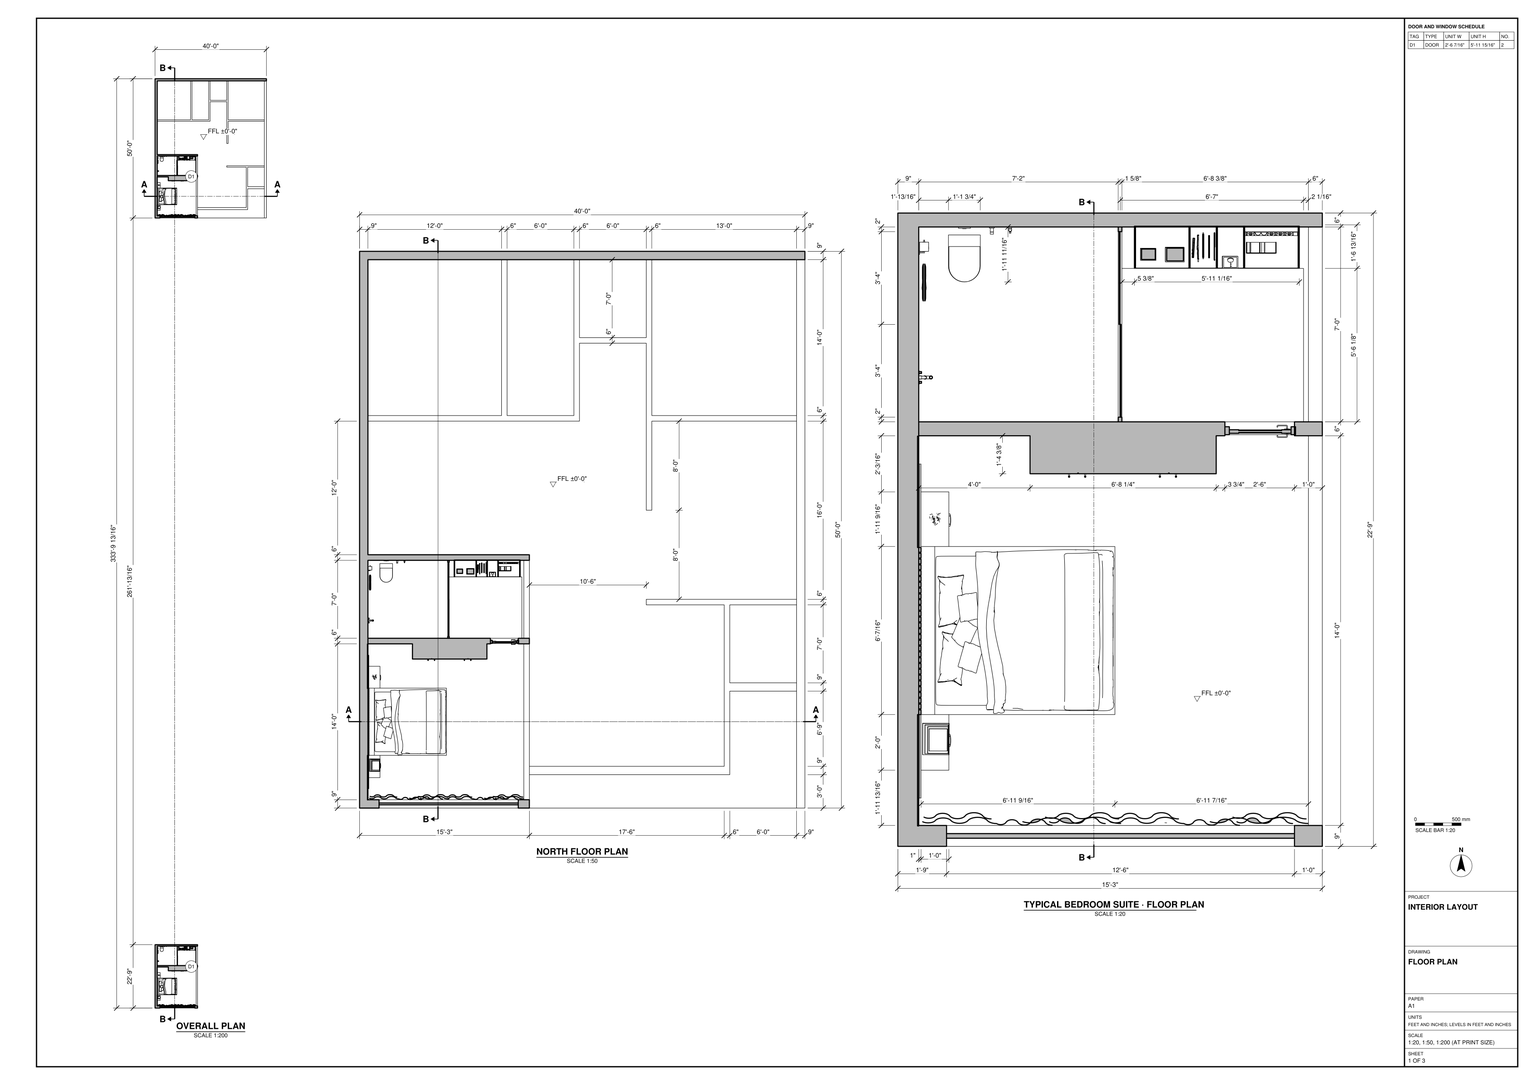
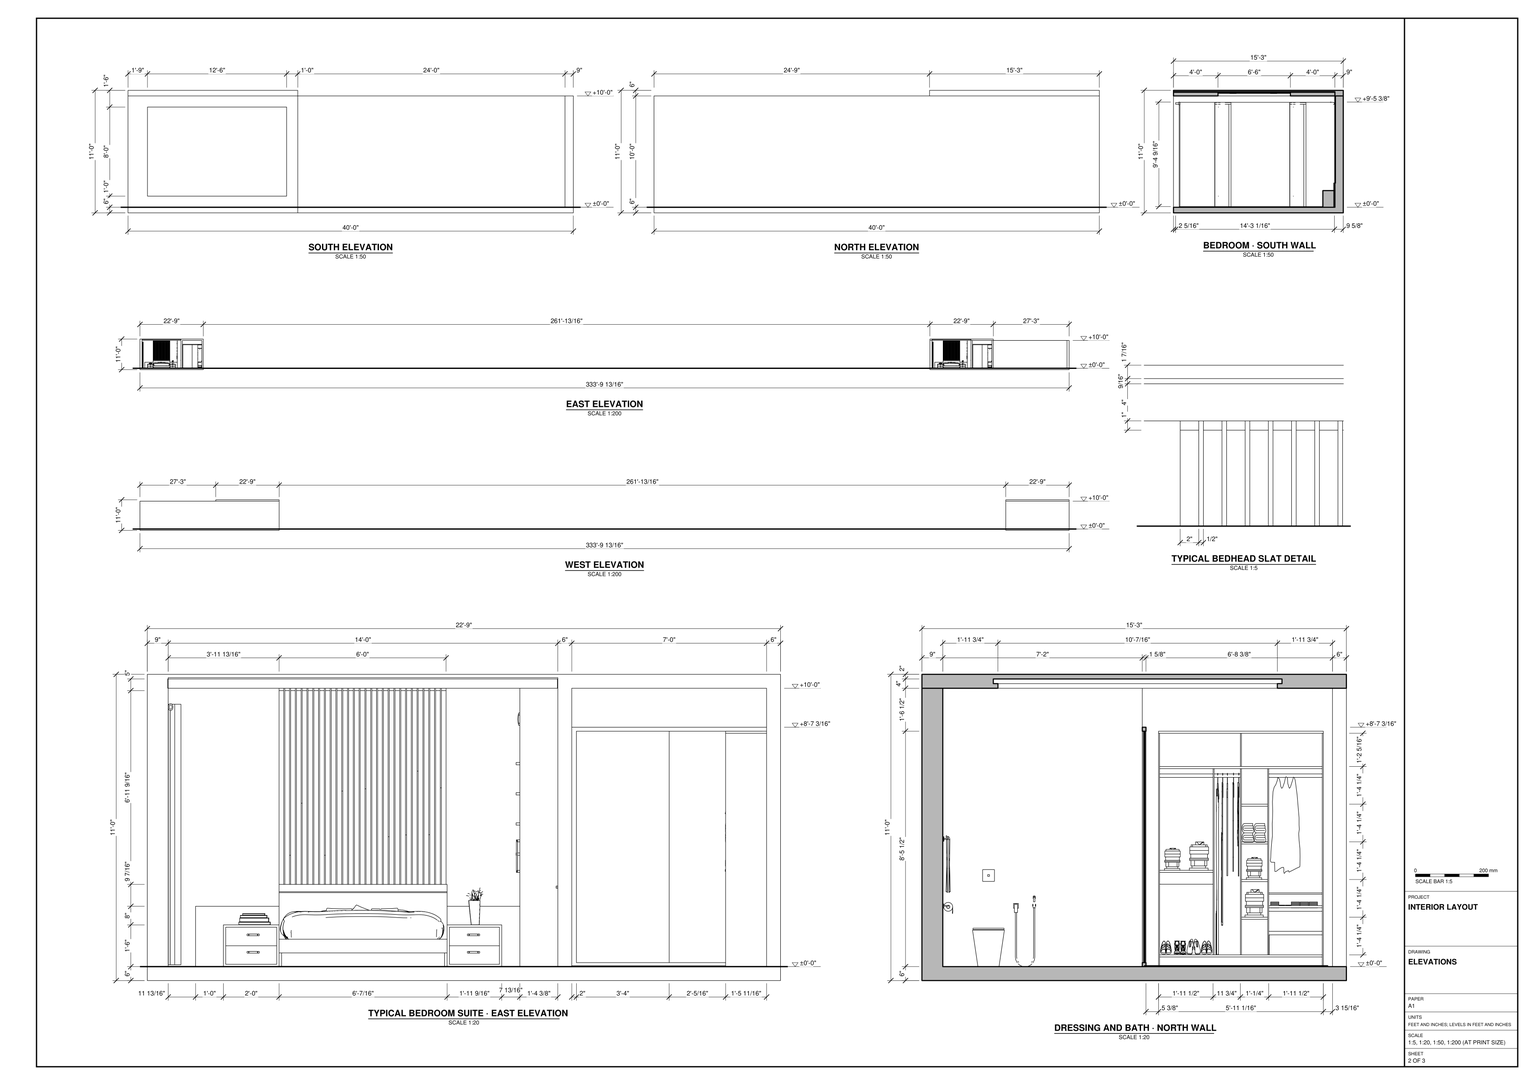
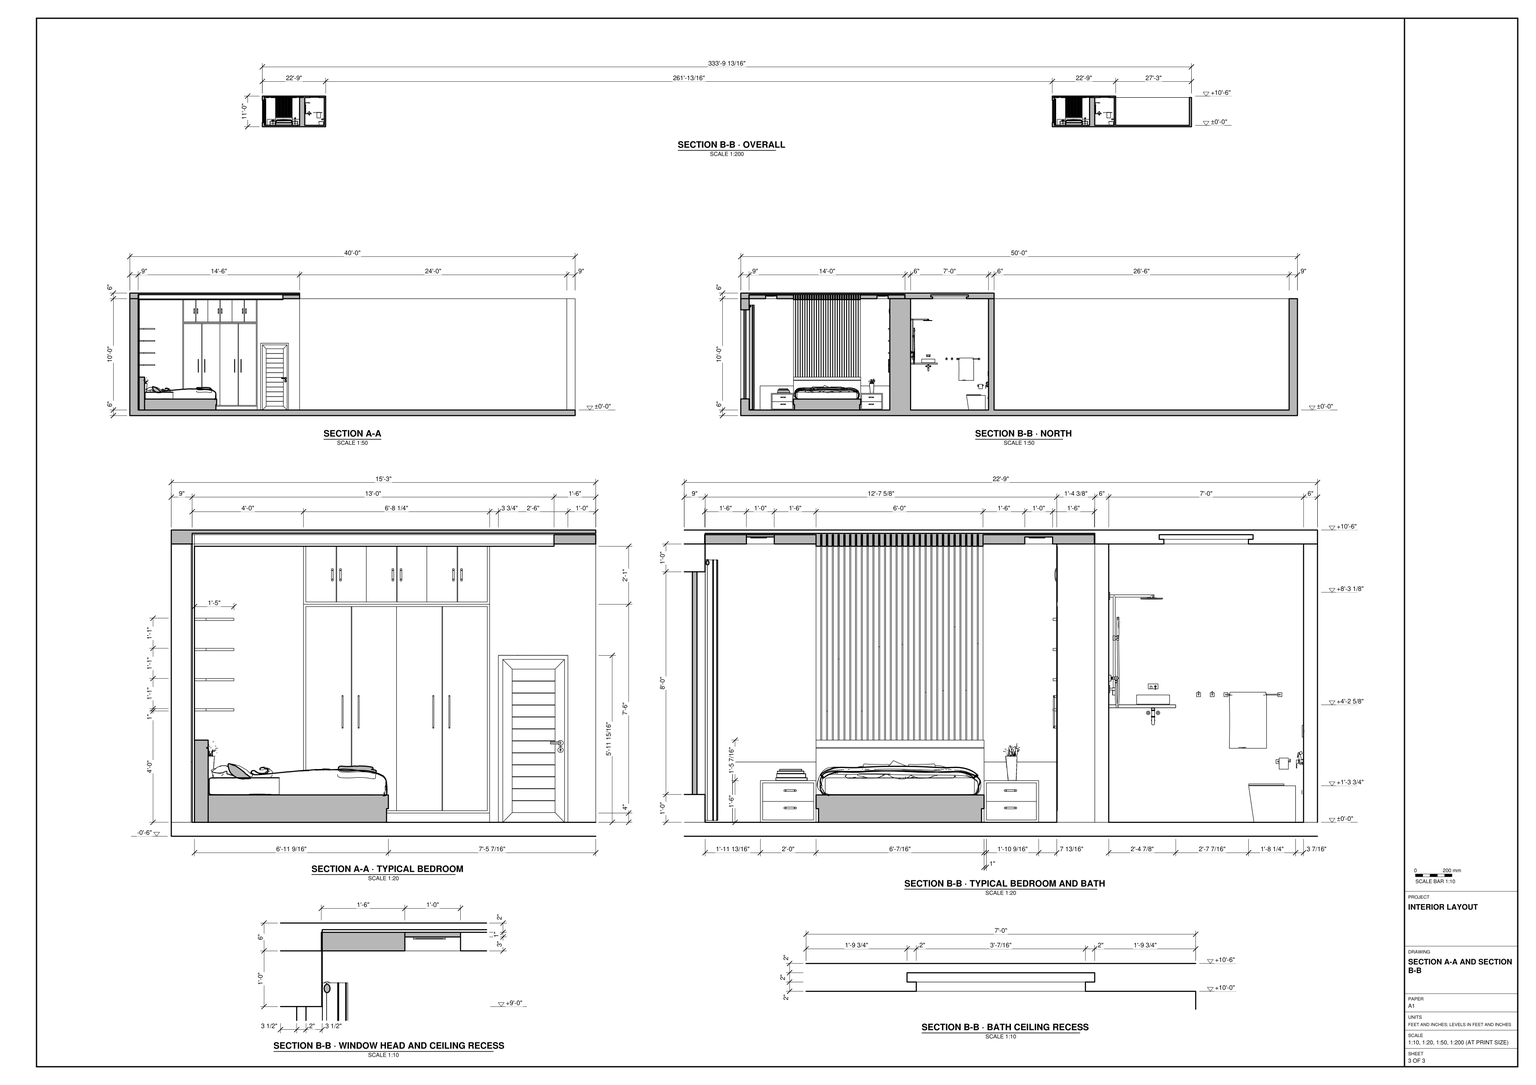
Work in feet and inches in SketchUp from task_files/diagram_01.pdf. Model the two locations shown on the overall plan: a furnished bedroom suite in the southwest corner of the 40'-0" by 50'-0" north floor layout, and a matching, separate suite to the south. Align their west walls and leave the intervening space clear. The complete model must measure 40'-0" along X, 333'-9 13/16" along Y and 11'-0" along Z. Use the single finished floor level of ±0'-0" at both locations.

Follow the north floor plan for the surrounding slab and wall layout. Use the enlarged suite plan, elevations and sections for the wall thicknesses, floor and roof slabs, ceiling recesses, bedroom window and door into the dressing area. In each suite, place the platform bed against the slatted bedhead, with a drawer unit on either side. Fit the bedroom wardrobe and overhead cupboards beside the door. Beyond the bedroom, separate the bath fixtures from the dressing bay and model the open wardrobe with its shelves, hanging spaces and drawers. Decor and loose items, including curtains, clothing, towels and plants, may be any suitable library components.

Keep shell elements such as walls, slabs and roof separate as groups or components. Group each furniture or joinery piece separately and use components for repeated parts. Save one SketchUp model as output_files/bedroom_suites_and_surrounding_north_floor_layout.skp.

# SketchUp Ruby script. Lengths in inches.
U = 1.inch
M = Sketchup.active_model
def pt(a) = Geom::Point3d.new(a.map { |v| v * U })
def face(e, loops, mat)
  f = e.add_face(loops[0].map { |a| pt(a) })
  loops[1..].each { |l| e.add_face(l.map { |a| pt(a) }).erase! }
  f.material = f.back_material = mat if mat
  f
end
# faces: each face lists its corners as indices into pts; further lists are holes
def faces(e, pts, list, mat = nil) = list.each { |f| face(e, (f[0].is_a?(Array) ? f : [f]).map { |l| l.map { |i| pts[i] } }, mat) }
# xy, xz, yz: faces in a plane at the given z, y or x. An outline is a flat list of corners, or four numbers for a rectangle; further outlines are holes
def ring(l) = l.size == 4 ? [[l[0], l[1]], [l[2], l[1]], [l[2], l[3]], [l[0], l[3]]] : l.each_slice(2).to_a
def flat(e, list, mat, &to3) = list.each { |f| face(e, (f[0].is_a?(Array) ? f : [f]).map { |l| ring(l).map { |u, v| to3.(u, v) } }, mat) }
def xy(e, z, list, mat = nil) = flat(e, list, mat) { |x, y| [x, y, z] }
def xz(e, y, list, mat = nil) = flat(e, list, mat) { |x, z| [x, y, z] }
def yz(e, x, list, mat = nil) = flat(e, list, mat) { |y, z| [x, y, z] }
def lines(e, pts, list) = list.each { |a, b| e.add_line(pt(pts[a]), pt(pts[b])) }
# prism: a flat outline (further loops are holes) pulled along v
def prism(e, loops, v, mat = nil)
  f = face(e, loops, mat); d = Geom::Vector3d.new(v.map { |x| x * U })
  f.pushpull(f.normal.samedirection?(d) ? d.length : -d.length)
end
def box(e, o, s, mat = nil) = prism(e, [[o, [o[0] + s[0], o[1], o[2]], [o[0] + s[0], o[1] + s[1], o[2]], [o[0], o[1] + s[1], o[2]]]], [0, 0, s[2]], mat)
def at(x, y, z, deg = 0) = Geom::Transformation.translation(pt([x, y, z])) * Geom::Transformation.rotation(ORIGIN, Z_AXIS, deg.degrees)
def axes(o, x, y, z) = Geom::Transformation.new([*x, 0, *y, 0, *z, 0, *pt(o).to_a, 1])
def part(name) = M.definitions.add(name)
# library, detail: a bought-in or finely detailed component or shape, given as its bounding box
def library(name, o, s) = part(name).tap { |d| box(d.entities, o, s) }
def detail(e, o, s) = box(e.add_group.entities, o, s)
def put(e, d, t, mat = nil) = e.add_instance(d, t).tap { |i| i.material = mat if mat }
def group(e, t, mat = nil) = e.add_group.tap { |g| g.transformation = t; g.material = mat if mat }.entities
root = M.entities
M.materials.add("0915 AP 7850 BANANA CREAM").color = [226, 212, 179]
M.materials.add("1833 AP 8596 CRYSTAL BEACH").color = [234, 228, 220]
M.materials.add("Carpet_Frieze_Low").color = [170, 156, 146]
M.materials.add("Carpet_Loop_Low").color = [201, 172, 127]
M.materials["Carpet_Loop_Low"].alpha = 0.3
M.materials.add("Emissive\#1").color = [251, 252, 224]
M.materials.add("Glass Bumpy 03 10cm").color = [188, 188, 188]
M.materials["Glass Bumpy 03 10cm"].alpha = 0.15
M.materials.add("Glass Safety Distorted 001").color = [249, 255, 239]
M.materials["Glass Safety Distorted 001"].alpha = 0.1
M.materials.add("Maquette Wood B01 12cm").color = [172, 139, 101]
M.materials.add("PDM_chrome").color = [38, 38, 38]
M.materials.add("Tiles Grey 13 135cm").color = [141, 141, 136]
M.materials.add("Tiles Marble White 03 180cm").color = [241, 241, 241]
M.materials.add("Tiles Patterned 07 80cm\#2").color = [154, 140, 117]
M.materials.add("W150Z669S75_Sabya 3 Gokul Pichwai-Khubanee").color = [172, 128, 96]
M.materials.add("[Aluminum]").color = [179, 179, 179]
c1 = part("Curtain panel")
p = [[17.625,0.0625,78.74],[17.625,0.0625,0],[18.27,0,0],[18.27,0,78.74],[18.92,0.0625,0],[18.92,0.0625,78.74],
  [17,0.25,78.74],[17,0.25,0],[19.55,0.25,0],[19.55,0.25,78.74],[16.43,0.56,78.74],[16.43,0.56,0],
  [20.12,0.56,0],[20.12,0.56,78.74],[6.31,0.6,78.74],[6.31,0.6,0],[6.8125,0.45,0],[6.8125,0.45,78.74],
  [7.33,0.4,0],[7.33,0.4,78.74],[7.86,0.45,0],[7.86,0.45,78.74],[8.36,0.6,0],[8.36,0.6,78.74],
  [5.85,0.85,78.74],[5.85,0.85,0],[8.82,0.85,0],[8.82,0.85,78.74],[15.92,0.97,78.74],[15.92,0.97,0],
  [20.625,0.97,0],[20.625,0.97,78.74],[5.44,1.18,78.74],[5.44,1.18,0],[9.23,1.18,0],[9.23,1.18,78.74],
  [15.51,1.48,78.74],[15.51,1.48,0],[21.04,1.48,0],[21.04,1.48,78.74],[5.11,1.59,78.74],[5.11,1.59,0],
  [9.5625,1.59,0],[9.5625,1.59,78.74],[14.93,2.55,78.74],[14.93,2.55,0],[15.2,2.04,0],[15.2,2.04,78.74],
  [21.34,2.04,0],[21.64,2.59,0],[21.64,2.59,78.74],[21.34,2.04,78.74],[4.63,2.47,78.74],[4.63,2.47,0],
  [4.86,2.04,0],[4.86,2.04,78.74],[9.81,2.04,0],[10.08,2.55,0],[10.08,2.55,78.74],[9.81,2.04,78.74],
  [4.32,2.85,78.74],[4.32,2.85,0],[10.44,2.99,0],[10.44,2.99,78.74],[14.57,2.99,78.74],[14.57,2.99,0],
  [22.03,3.0625,0],[22.03,3.0625,78.74],[0.85,2.85,78.74],[0.85,2.85,0],[1.22,3.15,0],[1.22,3.15,78.74],
  [3.95,3.15,78.74],[3.95,3.15,0],[10.89,3.35,0],[10.89,3.35,78.74],[14.125,3.35,78.74],[14.125,3.35,0],
  [22.5,3.45,0],[22.5,3.45,78.74],[1.65,3.375,0],[1.65,3.375,78.74],[3.53,3.375,78.74],[3.53,3.375,0],
  [2.11,3.52,0],[2.11,3.52,78.74],[3.07,3.52,78.74],[3.07,3.52,0],[11.39,3.625,0],[11.39,3.625,78.74],
  [13.62,3.625,78.74],[13.62,3.625,0],[2.59,3.5625,0],[2.59,3.5625,78.74],[23.04,3.74,0],[23.04,3.74,78.74],
  [11.9375,3.79,0],[11.9375,3.79,78.74],[13.07,3.79,78.74],[13.07,3.79,0],[23.63,3.92,0],[23.63,3.92,78.74],
  [12.51,3.85,0],[12.51,3.85,78.74],[24.25,3.98,0],[24.25,3.98,78.74],[5.51,1.25,0],[5.9,0.93,0],
  [4.95,2.09,0],[5.1875,1.64,0],[6.35,0.69,0],[6.83,0.55,0],[7.33,0.5,0],[7.84,0.55,0],
  [8.32,0.69,0],[8.77,0.93,0],[9.16,1.25,0],[9.48,1.64,0],[9.72,2.09,0],[10,2.61,0],
  [10.375,3.0625,0],[10.83,3.4375,0],[17.64,0.16,0],[18.27,0.1,0],[11.35,3.71,0],[11.92,3.89,0],
  [12.51,3.94,0],[13.09,3.89,0],[20.56,1.04,0],[20.96,1.53,0],[13.66,3.71,0],[14.18,3.4375,0],
  [14.64,3.0625,0],[15.01,2.61,0],[15.29,2.09,0],[15.59,1.53,0],[15.99,1.04,0],[16.48,0.64,0],
  [17.04,0.34,0],[18.9,0.16,0],[19.51,0.34,0],[20.07,0.64,0],[21.26,2.09,0],[21.56,2.64,0],
  [21.96,3.13,0],[22.45,3.53,0],[23,3.83,0],[23.61,4.01,0],[24.24,4.08,0]]
faces(c1.entities,p,[[0,1,2,3],[3,2,4,5],[6,7,1,0],[5,4,8,9],[10,11,7,6],[9,8,12,13],[14,15,16,17],[17,16,18,19],
  [19,18,20,21],[21,20,22,23],[24,25,15,14],[23,22,26,27],[28,29,11,10],[13,12,30,31],[32,33,25,24],[27,26,34,35],
  [36,37,29,28],[31,30,38,39],[40,41,33,32],[35,34,42,43],[44,45,46,37,36,47],[39,38,48,49,50,51],[52,53,54,41,40,55],[43,42,56,57,58,59],
  [60,61,53,52],[58,57,62,63],[64,65,45,44],[50,49,66,67],[68,69,70,71],[72,73,61,60],[63,62,74,75],[76,77,65,64],
  [67,66,78,79],[71,70,80,81],[82,83,73,72],[81,80,84,85],[86,87,83,82],[75,74,88,89],[90,91,77,76],[85,84,92,93],
  [93,92,87,86],[79,78,94,95],[89,88,96,97],[98,99,91,90],[95,94,100,101],[97,96,102,103],[103,102,99,98],[101,100,104,105]])
lines(c1.entities,p,[[106,107],[108,109],[109,106],[107,110],[110,111],[111,112],[112,113],[113,114],[114,115],[115,116],[116,117],[117,118],
  [118,119],[119,120],[120,121],[122,123],[121,124],[124,125],[125,126],[126,127],[128,129],[127,130],[130,131],[131,132],
  [132,133],[133,134],[134,135],[135,136],[136,137],[137,138],[138,122],[123,139],[139,140],[140,141],[141,128],[129,142],
  [142,143],[143,144],[144,145],[145,146],[146,147],[147,148],[148,104]])
c2 = part("Curtain rod section")
yz(c2.entities,0,[[1.55,0.61,1.31,0.64,1.08,0.73,0.88,0.88,0.73,1.08,0.64,1.31,0.61,1.55,0.64,1.79,0.73,2.02,0.88,2.22,1.08,2.37,1.31,2.46,1.55,2.49,1.79,2.46,2.02,2.37,2.22,2.22,2.37,2.02,2.46,1.79,2.49,1.55,2.46,1.31,2.37,1.08,2.22,0.88,2.02,0.73,1.79,0.64]])
yz(c2.entities,2.36,[[[1.55,0,1.15,0.05,0.78,0.21,0.45,0.45,0.21,0.78,0.05,1.15,0,1.55,0.05,1.95,0.21,2.33,0.45,2.65,0.78,2.89,1.15,3.05,1.55,3.1,1.95,3.05,2.33,2.89,2.65,2.65,2.89,2.33,3.05,1.95,3.1,1.55,3.05,1.15,2.89,0.78,2.65,0.45,2.33,0.21,1.95,0.05],[1.55,0.61,1.79,0.64,2.02,0.73,2.22,0.88,2.37,1.08,2.46,1.31,2.49,1.55,2.46,1.79,2.37,2.02,2.22,2.22,2.02,2.37,1.79,2.46,1.55,2.49,1.31,2.46,1.08,2.37,0.88,2.22,0.73,2.02,0.64,1.79,0.61,1.55,0.64,1.31,0.73,1.08,0.88,0.88,1.08,0.73,1.31,0.64]]])
yz(c2.entities,3.15,[[[1.55,0,1.95,0.05,2.33,0.21,2.65,0.45,2.89,0.78,3.05,1.15,3.1,1.55,3.05,1.95,2.89,2.33,2.65,2.65,2.33,2.89,1.95,3.05,1.55,3.1,1.15,3.05,0.78,2.89,0.45,2.65,0.21,2.33,0.05,1.95,0,1.55,0.05,1.15,0.21,0.78,0.45,0.45,0.78,0.21,1.15,0.05],[1.55,0.61,1.31,0.64,1.08,0.73,0.88,0.88,0.73,1.08,0.64,1.31,0.61,1.55,0.64,1.79,0.73,2.02,0.88,2.22,1.08,2.37,1.31,2.46,1.55,2.49,1.79,2.46,2.02,2.37,2.22,2.22,2.37,2.02,2.46,1.79,2.49,1.55,2.46,1.31,2.37,1.08,2.22,0.88,2.02,0.73,1.79,0.64]]])
yz(c2.entities,61.24,[[1.55,0.61,1.79,0.64,2.02,0.73,2.22,0.88,2.37,1.08,2.46,1.31,2.49,1.55,2.46,1.79,2.37,2.02,2.22,2.22,2.02,2.37,1.79,2.46,1.55,2.49,1.31,2.46,1.08,2.37,0.88,2.22,0.73,2.02,0.64,1.79,0.61,1.55,0.64,1.31,0.73,1.08,0.88,0.88,1.08,0.73,1.31,0.64]])
p = [[2.36,1.15,0.05],[2.36,1.55,0],[3.15,1.55,0],[3.15,1.15,0.05],[2.36,1.95,0.05],[3.15,1.95,0.05],
  [2.36,0.78,0.21],[3.15,0.78,0.21],[2.36,2.33,0.21],[3.15,2.33,0.21],[2.36,0.45,0.45],[3.15,0.45,0.45],
  [2.36,2.65,0.45],[3.15,2.65,0.45],[2.36,0.21,0.78],[3.15,0.21,0.78],[2.36,2.89,0.78],[3.15,2.89,0.78],
  [2.36,1.31,0.64],[2.36,1.08,0.73],[0,1.08,0.73],[0,1.31,0.64],[3.15,1.31,0.64],[3.15,1.08,0.73],
  [61.24,1.31,0.64],[61.24,1.08,0.73],[2.36,1.55,0.61],[0,1.55,0.61],[3.15,1.55,0.61],[61.24,1.55,0.61],
  [2.36,1.79,0.64],[0,1.79,0.64],[3.15,1.79,0.64],[61.24,1.79,0.64],[2.36,2.02,0.73],[0,2.02,0.73],
  [3.15,2.02,0.73],[61.24,2.02,0.73],[2.36,0.88,0.88],[0,0.88,0.88],[3.15,0.88,0.88],[61.24,0.88,0.88],
  [2.36,2.22,0.88],[0,2.22,0.88],[3.15,2.22,0.88],[61.24,2.22,0.88],[2.36,0.05,1.15],[3.15,0.05,1.15],
  [2.36,3.05,1.15],[3.15,3.05,1.15],[2.36,0.73,1.08],[0,0.73,1.08],[3.15,0.73,1.08],[61.24,0.73,1.08],
  [2.36,2.37,1.08],[0,2.37,1.08],[3.15,2.37,1.08],[61.24,2.37,1.08],[2.36,0,1.55],[3.15,0,1.55],
  [2.36,0.64,1.31],[0,0.64,1.31],[3.15,0.64,1.31],[61.24,0.64,1.31],[2.36,2.46,1.31],[0,2.46,1.31],
  [3.15,2.46,1.31],[61.24,2.46,1.31],[2.36,3.1,1.55],[3.15,3.1,1.55],[2.36,0.61,1.55],[0,0.61,1.55],
  [3.15,0.61,1.55],[61.24,0.61,1.55],[2.36,2.49,1.55],[0,2.49,1.55],[3.15,2.49,1.55],[61.24,2.49,1.55],
  [2.36,0.05,1.95],[3.15,0.05,1.95],[2.36,0.64,1.79],[0,0.64,1.79],[3.15,0.64,1.79],[61.24,0.64,1.79],
  [2.36,2.46,1.79],[0,2.46,1.79],[3.15,2.46,1.79],[61.24,2.46,1.79],[2.36,3.05,1.95],[3.15,3.05,1.95],
  [2.36,0.73,2.02],[0,0.73,2.02],[3.15,0.73,2.02],[61.24,0.73,2.02],[2.36,2.37,2.02],[0,2.37,2.02],
  [3.15,2.37,2.02],[61.24,2.37,2.02],[2.36,0.21,2.33],[3.15,0.21,2.33],[2.36,0.88,2.22],[0,0.88,2.22],
  [3.15,0.88,2.22],[61.24,0.88,2.22],[2.36,2.22,2.22],[0,2.22,2.22],[3.15,2.22,2.22],[61.24,2.22,2.22],
  [2.36,2.89,2.33],[3.15,2.89,2.33],[2.36,1.08,2.37],[0,1.08,2.37],[3.15,1.08,2.37],[61.24,1.08,2.37],
  [2.36,2.02,2.37],[0,2.02,2.37],[3.15,2.02,2.37],[61.24,2.02,2.37],[2.36,0.45,2.65],[3.15,0.45,2.65],
  [2.36,2.65,2.65],[3.15,2.65,2.65],[2.36,1.31,2.46],[0,1.31,2.46],[3.15,1.31,2.46],[61.24,1.31,2.46],
  [2.36,1.79,2.46],[0,1.79,2.46],[3.15,1.79,2.46],[61.24,1.79,2.46],[2.36,1.55,2.49],[0,1.55,2.49],
  [3.15,1.55,2.49],[61.24,1.55,2.49],[2.36,0.78,2.89],[3.15,0.78,2.89],[2.36,2.33,2.89],[3.15,2.33,2.89],
  [2.36,1.15,3.05],[3.15,1.15,3.05],[2.36,1.95,3.05],[3.15,1.95,3.05],[2.36,1.55,3.1],[3.15,1.55,3.1]]
faces(c2.entities,p,[[0,1,2,3],[1,4,5,2],[6,0,3,7],[4,8,9,5],[10,6,7,11],[8,12,13,9],[14,10,11,15],[12,16,17,13],
  [18,19,20,21],[19,18,22,23],[24,25,23,22],[26,18,21,27],[18,26,28,22],[29,24,22,28],[30,26,27,31],[26,30,32,28],
  [33,29,28,32],[34,30,31,35],[30,34,36,32],[37,33,32,36],[19,38,39,20],[38,19,23,40],[25,41,40,23],[42,34,35,43],
  [34,42,44,36],[45,37,36,44],[46,14,15,47],[16,48,49,17],[38,50,51,39],[50,38,40,52],[41,53,52,40],[54,42,43,55],
  [42,54,56,44],[57,45,44,56],[58,46,47,59],[50,60,61,51],[60,50,52,62],[53,63,62,52],[64,54,55,65],[54,64,66,56],
  [67,57,56,66],[48,68,69,49],[60,70,71,61],[70,60,62,72],[63,73,72,62],[74,64,65,75],[64,74,76,66],[77,67,66,76],
  [78,58,59,79],[70,80,81,71],[80,70,72,82],[73,83,82,72],[84,74,75,85],[74,84,86,76],[87,77,76,86],[68,88,89,69],
  [80,90,91,81],[90,80,82,92],[83,93,92,82],[94,84,85,95],[84,94,96,86],[97,87,86,96],[98,78,79,99],[90,100,101,91],
  [100,90,92,102],[93,103,102,92],[104,94,95,105],[94,104,106,96],[107,97,96,106],[88,108,109,89],[100,110,111,101],[110,100,102,112],
  [103,113,112,102],[114,104,105,115],[104,114,116,106],[117,107,106,116],[118,98,99,119],[108,120,121,109],[110,122,123,111],[122,110,112,124],
  [113,125,124,112],[126,114,115,127],[114,126,128,116],[129,117,116,128],[122,130,131,123],[130,122,124,132],[125,133,132,124],[130,126,127,131],
  [126,130,132,128],[133,129,128,132],[134,118,119,135],[120,136,137,121],[138,134,135,139],[136,140,141,137],[142,138,139,143],[140,142,143,141]])
c3 = part("Curtain rod assembly")
put(c3.entities,c2,axes([3.125,-0.76,-71.54],[0,0,1.25313],[0,1.25313,0],[-1.25313,0,0]))
put(c3.entities,c2,axes([3.125,3.125,81],[0,0,-1.25313],[0,-1.25313,0],[-1.25313,0,0]))
c4 = part("Group\#57")
put(c4.entities,c1,axes([-0.76,0,0],[0.8979,0,0],[0,1,0],[0,0,1]),"Carpet_Frieze_Low")
put(c4.entities,c1,axes([37.23,0,0],[0.9782,0,0],[0,1,0],[0,0,1]),"Carpet_Frieze_Low")
c5 = part("curtain2")
p = [[59.99,12.8,78.74],[59.99,12.8,-38.1875],[60.15,12.52,-38.1875],[60.15,12.52,78.74],[66.72,13.7,-38.1875],[66.72,13.7,78.74],
  [73.91,13.97,78.74],[73.91,13.97,-38.1875],[49.31,14.13,-38.1875],[49.31,14.13,78.74],[2.67,12.52,-38.1875],[2.67,12.52,78.74],
  [-8.17,14.13,-38.1875],[-8.17,14.13,78.74],[2.51,12.8,78.74],[2.51,12.8,-38.1875],[16.42,13.97,78.74],[16.42,13.97,-38.1875],
  [9.24,13.7,-38.1875],[9.24,13.7,78.74]]
lines(c5.entities,p,[[0,1],[2,3],[4,5],[6,7],[8,9],[10,11],[12,13],[14,15],[16,17],[18,19]])
put(c5.entities,c1,axes([64.94,10.15,-38.1875],[0.73,0,0],[0,1,0],[0,0,1.485]),"Carpet_Loop_Low")
put(c5.entities,c1,axes([48.6875,11.28,-38.1875],[0.73,0,0],[0,1,0],[0,0,1.485]),"Carpet_Loop_Low")
put(c5.entities,c1,axes([25.83,10.15,-38.1875],[0.96815,0,0],[0,1,0],[0,0,1.485]),"Carpet_Loop_Low")
put(c5.entities,c1,axes([56.28,10.09,-38.1875],[1.28298,0,0],[0,1,0],[0,0,1.485]),"Carpet_Loop_Low")
put(c5.entities,c3,axes([25.47,12.88,78.42],[0,0,-0.798],[0,0.798,0],[0.798,0,0]))
put(c5.entities,c1,axes([7.46,10.15,-38.1875],[0.73,0,0],[0,1,0],[0,0,1.485]),"Carpet_Loop_Low")
put(c5.entities,c1,axes([-1.2,10.09,-38.1875],[1.28298,0,0],[0,1,0],[0,0,1.485]),"Carpet_Loop_Low")
put(c5.entities,c1,axes([-8.79,11.28,-38.1875],[0.73,0,0],[0,1,0],[0,0,1.485]),"Carpet_Loop_Low")
put(c5.entities,c1,axes([-31.65,10.15,-38.1875],[0.96815,0,0],[0,1,0],[0,0,1.485]),"Carpet_Loop_Low")
put(c5.entities,c4,axes([27.05,7.18,-38.1875],[0.98,0,0],[0,1,0],[0,0,1.485]))
put(c5.entities,c4,axes([-30.43,7.18,-38.1875],[0.98,0,0],[0,1,0],[0,0,1.485]))
c6 = part("Curtains")
put(c6.entities,c5,axes([31.62,15.375,38.1875],[1,0,0],[0,-1,0],[0,0,1]))
c7 = part("Bar")
prism(c7.entities,[[[0,0.49,0.31],[0,0.5,0.25],[0,0.49,0.19],[0,0.47,0.125],[0,0.43,0.07],[0,0.375,0.03],[0,0.31,0.01],[0,0.25,0],[0,0.19,0.01],[0,0.125,0.03],[0,0.07,0.07],[0,0.03,0.125],[0,0.01,0.19],[0,0,0.25],[0,0.01,0.31],[0,0.03,0.375],[0,0.07,0.43],[0,0.125,0.47],[0,0.19,0.49],[0,0.25,0.5],[0,0.31,0.49],[0,0.375,0.47],[0,0.43,0.43],[0,0.47,0.375]]],[11.5,0,0],"PDM_chrome")
c8 = part("End")
xy(c8.entities,0,[[0,0.25,0.875,1.5]],"PDM_chrome")
xy(c8.entities,0.5,[[0,0.25,0.875,1.5]],"PDM_chrome")
xz(c8.entities,1.5,[[0,0,0.875,0.5]],"PDM_chrome")
yz(c8.entities,0,[[0.25,0,0.19,0.01,0.125,0.03,0.07,0.07,0.03,0.125,0.01,0.19,0,0.25,0.01,0.31,0.03,0.375,0.07,0.43,0.125,0.47,0.19,0.49,0.25,0.5,1.5,0.5,1.5,0]],"PDM_chrome")
yz(c8.entities,0.25,[[0.25,0,0.31,0.01,0.375,0.03,0.43,0.07,0.47,0.125,0.49,0.19,0.5,0.25,0.49,0.31,0.47,0.375,0.43,0.43,0.375,0.47,0.31,0.49,0.25,0.5,0.19,0.49,0.125,0.47,0.07,0.43,0.03,0.375,0.01,0.31,0,0.25,0.01,0.19,0.03,0.125,0.07,0.07,0.125,0.03,0.19,0.01]],"PDM_chrome")
yz(c8.entities,0.875,[[0.25,0,1.5,0,1.5,0.5,0.25,0.5,0.31,0.49,0.375,0.47,0.43,0.43,0.47,0.375,0.49,0.31,0.5,0.25,0.49,0.19,0.47,0.125,0.43,0.07,0.375,0.03,0.31,0.01]],"PDM_chrome")
p = [[0.25,0.125,0.03],[0,0.125,0.03],[0,0.19,0.01],[0.25,0.19,0.01],[0.25,0.07,0.07],[0,0.07,0.07],
  [0,0.25,0],[0.25,0.25,0],[0.875,0.25,0],[0.875,0.31,0.01],[0.25,0.31,0.01],[0.875,0.375,0.03],
  [0.25,0.375,0.03],[0.875,0.43,0.07],[0.25,0.43,0.07],[0.25,0.01,0.19],[0,0.01,0.19],[0,0.03,0.125],
  [0.25,0.03,0.125],[0.875,0.47,0.125],[0.25,0.47,0.125],[0.875,0.49,0.19],[0.25,0.49,0.19],[0.25,0.01,0.31],
  [0,0.01,0.31],[0,0,0.25],[0.25,0,0.25],[0.875,0.5,0.25],[0.25,0.5,0.25],[0.875,0.49,0.31],
  [0.25,0.49,0.31],[0.25,0.03,0.375],[0,0.03,0.375],[0.875,0.47,0.375],[0.25,0.47,0.375],[0.25,0.07,0.43],
  [0,0.07,0.43],[0.25,0.125,0.47],[0,0.125,0.47],[0.875,0.43,0.43],[0.25,0.43,0.43],[0.875,0.375,0.47],
  [0.25,0.375,0.47],[0.25,0.19,0.49],[0,0.19,0.49],[0.25,0.25,0.5],[0,0.25,0.5],[0.875,0.31,0.49],
  [0.875,0.25,0.5],[0.25,0.31,0.49]]
faces(c8.entities,p,[[0,1,2,3],[4,5,1,0],[3,2,6,7],[8,9,10,7],[9,11,12,10],[11,13,14,12],[15,16,17,18],[18,17,5,4],
  [13,19,20,14],[19,21,22,20],[23,24,25,26],[26,25,16,15],[21,27,28,22],[27,29,30,28],[31,32,24,23],[29,33,34,30],
  [35,36,32,31],[37,38,36,35],[33,39,40,34],[39,41,42,40],[43,44,38,37],[45,46,44,43],[47,48,45,49],[41,47,49,42]],"PDM_chrome")
c9 = part("Drawer Pull")
put(c9.entities,c7,axes([0.25,0,0],[1.18,0,0],[0,1,0],[0,0,1]),"PDM_chrome")
put(c9.entities,c8,at(0,0,0))
put(c9.entities,c8,axes([14.07,0,0],[-1,0,0],[0,1,0],[0,0,1]),"PDM_chrome")
c10 = part("handle")
put(c10.entities,c9,at(0,0,0),"PDM_chrome")
c11 = library("Handle_06.skp",[-2.68,-0.84,-0.37],[5.36,0.84,0.74])
c12 = library("suit+cabinet,+wardrop",[0,-1.33,0],[110.24,29.21,78.74])
c13 = part("WALL+ART-00")
g1 = group(c13.entities,at(0,0,0))
box(g1,[0,0,0],[98.79,72.84,0.29])
c14 = library("Bathroom",[1.26,0,0],[40.08,46.34,56.49])
c15 = library("Shower Raindance Connect",[1.71,-11.67,0],[20.76,23.22,49.85])
c16 = library("washbasin",[122.49,213.42,-11.07],[43.31,15.75,26.44])
c17 = library("Door+80x210",[17.88,40.74,0],[31.52,6.14,82.69])
c18 = library("Omni Light",[-12,-12,-12],[24,24,24])
c19 = library("Group\#1",[-0.5,0,0],[174.5,168,124])
c20 = part("Group\#43")
xy(c20.entities,0,[[0,0,2,84]],"[Aluminum]")
xy(c20.entities,2,[[0.5,2,1,42],[1,42,1.5,82]])
xy(c20.entities,2,[[0,2,0.5,2,0.5,42,1,42,1,82,0,82],[1,2,2,2,2,82,1.5,82,1.5,42,1,42]],"[Aluminum]")
xy(c20.entities,118,[[0.5,2,1,42],[1,42,1.5,82]])
xy(c20.entities,118,[[0,2,0,82,1,82,1,42,0.5,42,0.5,2],[1,2,1,42,1.5,42,1.5,82,2,82,2,2]],"[Aluminum]")
xy(c20.entities,120,[[0,0,2,84]],"[Aluminum]")
xz(c20.entities,0,[[0,0,2,120]],"[Aluminum]")
xz(c20.entities,2,[[0,2,0.5,118],[0.5,2,1,118],[1,2,2,118]])
xz(c20.entities,42,[[0.5,2,1,118],[1,2,1.5,118]])
xz(c20.entities,82,[[1,2,1.5,118],[1.5,2,2,118]])
xz(c20.entities,82,[[0,2,1,118]],"[Aluminum]")
xz(c20.entities,84,[[0,0,2,120]])
yz(c20.entities,0,[[[0,0,84,120],[2,2,82,118]]],"[Aluminum]")
yz(c20.entities,0.5,[[2,2,42,118]],"Glass Bumpy 03 10cm")
yz(c20.entities,1,[[2,2,42,118],[42,2,82,118]],"Glass Bumpy 03 10cm")
yz(c20.entities,1.5,[[42,2,82,118]],"Glass Bumpy 03 10cm")
yz(c20.entities,2,[[[0,0,84,120],[2,2,82,118]]],"[Aluminum]")
xy(root,-6,[[0,0,183,273],[0,3405.8125,480,4005.8125]])
xy(root,0,[[177,9,183,177],[95,183,177,267],[177,183,183,267],[183,3405.8125,471,3405.8125,471,3531.8125,399,3531.8125,399,3441.8125,183,3441.8125],[471,3405.8125,480,3996.8125],
  [177,3414.8125,183,3582.8125],[183,3441.8125,399,3441.8125,399,3531.8125,471,3531.8125,471,3540.8125,399,3540.8125,399,3624.8125,471,3624.8125,471,3630.8125,309,3630.8125,309,3624.8125,393,3624.8125,393,3450.8125,183,3450.8125],[183,3450.8125,393,3450.8125,393,3624.8125,309,3624.8125,309,3630.8125,471,3630.8125,471,3822.8125,315,3822.8125,315,3726.8125,309,3726.8125,309,3906.8125,237,3906.8125,237,3822.8125,9,3822.8125,9,3678.8125,183,3678.8125],[399,3540.8125,471,3624.8125],[95,3588.8125,177,3672.8125],
  [177,3588.8125,183,3672.8125],[309,3726.8125,315,3726.8125,315,3822.8125,471,3822.8125,471,3828.8125,315,3828.8125,315,3996.8125,309,3996.8125,309,3912.8125,237,3912.8125,237,3996.8125,231,3996.8125,231,3828.8125,159,3828.8125,159,3996.8125,153,3996.8125,153,3828.8125,9,3828.8125,9,3822.8125,237,3822.8125,237,3906.8125,309,3906.8125],[9,3828.8125,153,3996.8125],[159,3828.8125,231,3996.8125],[315,3828.8125,471,3996.8125],
  [237,3912.8125,309,3996.8125]])
xy(root,0,[[9,183,95,267],[9,3588.8125,95,3672.8125]],"Tiles Grey 13 135cm")
xy(root,0,[[9,9,177,9,177,177,171,177,171,183,141,183,141,177,137.25,177,137.25,160.625,57,160.625,57,177,9,177],[9,3414.8125,177,3414.8125,177,3582.8125,171,3582.8125,171,3588.8125,141,3588.8125,141,3582.8125,137.25,3582.8125,137.25,3566.4375,57,3566.4375,57,3582.8125,9,3582.8125]],"Tiles Marble White 03 180cm")
xy(root,5,[[77.5625,160.625,77.86,160.92],[116.6875,160.625,116.99,160.92],[77.5625,3566.4375,77.86,3566.74],[116.6875,3566.4375,116.99,3566.74]])
xy(root,12,[[21,0,171,3.5],[21,3.5,171,5.5],[21,5.5,171,9],[21,3405.8125,171,3409.3125],[21,3409.3125,171,3411.3125],
  [21,3411.3125,171,3414.8125]])
xy(root,48,[[9,159,9,177,27,177,27,171,15,171,15,159],[9,3564.8125,9,3582.8125,27,3582.8125,27,3576.8125,15,3576.8125,15,3564.8125]],"1833 AP 8596 CRYSTAL BEACH")
xy(root,49,[[9,159,15,159,15,171,27,171,27,177,9,177],[9,3564.8125,15,3564.8125,15,3576.8125,27,3576.8125,27,3582.8125,9,3582.8125]],"1833 AP 8596 CRYSTAL BEACH")
xy(root,61,[[9,159,9,177,27,177,27,171,15,171,15,159],[9,3564.8125,9,3582.8125,27,3582.8125,27,3576.8125,15,3576.8125,15,3564.8125]],"1833 AP 8596 CRYSTAL BEACH")
xy(root,62,[[9,159,15,159,15,171,27,171,27,177,9,177],[9,3564.8125,15,3564.8125,15,3576.8125,27,3576.8125,27,3582.8125,9,3582.8125]],"1833 AP 8596 CRYSTAL BEACH")
xy(root,72,[[141,177,171,183],[141,3582.8125,171,3588.8125]],"W150Z669S75_Sabya 3 Gokul Pichwai-Khubanee")
xy(root,74,[[9,159,9,177,27,177,27,171,15,171,15,159],[9,3564.8125,9,3582.8125,27,3582.8125,27,3576.8125,15,3576.8125,15,3564.8125]],"1833 AP 8596 CRYSTAL BEACH")
xy(root,75,[[9,159,15,159,15,171,27,171,27,177,9,177],[9,3564.8125,15,3564.8125,15,3576.8125,27,3576.8125,27,3582.8125,9,3582.8125]],"1833 AP 8596 CRYSTAL BEACH")
xy(root,87,[[9,159,9,177,27,177,27,171,15,171,15,159],[9,3564.8125,9,3582.8125,27,3582.8125,27,3576.8125,15,3576.8125,15,3564.8125]],"1833 AP 8596 CRYSTAL BEACH")
xy(root,88,[[9,159,15,159,15,171,27,171,27,177,9,177],[9,3564.8125,15,3564.8125,15,3576.8125,27,3576.8125,27,3582.8125,9,3582.8125]],"1833 AP 8596 CRYSTAL BEACH")
xy(root,93,[[77.5625,160.625,77.86,160.92],[116.6875,160.625,116.99,160.92],[77.5625,3566.4375,77.86,3566.74],[116.6875,3566.4375,116.99,3566.74]])
xy(root,95,[[71.04,160.625,71.34,160.92],[97.125,160.625,97.43,160.92],[123.21,160.625,123.51,160.92],[71.04,3566.4375,71.34,3566.74],[97.125,3566.4375,97.43,3566.74],
  [123.21,3566.4375,123.51,3566.74]])
xy(root,108,[[21,0,171,3.5],[21,3.5,171,5.5],[21,5.5,171,9],[21,3405.8125,171,3409.3125],[21,3409.3125,171,3411.3125],
  [21,3411.3125,171,3414.8125]])
xy(root,119,[[71.04,160.625,71.34,160.92],[97.125,160.625,97.43,160.92],[123.21,160.625,123.51,160.92],[71.04,3566.4375,71.34,3566.74],[97.125,3566.4375,97.43,3566.74],
  [123.21,3566.4375,123.51,3566.74]])
xy(root,120,[[0,0,9,273],[57,160.625,137.25,177],[[9,183,177,267],[32.77,206.77,153.23,243.23]],[177,183,183,267],[9,267,177,273],
  [0,3405.8125,9,3678.8125],[9,3405.8125,183,3414.8125],[57,3566.4375,137.25,3582.8125],[9,3582.8125,183,3588.8125],[[9,3588.8125,177,3672.8125],[32.77,3612.59,153.23,3649.04]],
  [177,3588.8125,183,3672.8125],[9,3672.8125,177,3678.8125],[177,3672.8125,183,3678.8125],[0,3678.8125,9,3678.8125,9,3996.8125,480,3996.8125,480,4005.8125,0,4005.8125]])
xy(root,122,[[30.77,204.77,155.23,206.77],[30.77,206.77,32.77,245.23],[153.23,206.77,155.23,243.23],[32.77,243.23,155.23,245.23],[30.77,3610.59,155.23,3612.59],
  [30.77,3612.59,32.77,3651.04],[153.23,3612.59,155.23,3649.04],[32.77,3649.04,155.23,3651.04]])
xy(root,124,[[30.77,204.77,155.23,245.23],[30.77,3610.59,155.23,3651.04]])
xy(root,124.5625,[[9,9,183,177],[9,3414.8125,183,3582.8125]])
xy(root,126,[[0,0,183,273],[0,3405.8125,183,3678.8125]])
xz(root,0,[[[0,-6,183,120],[21,12,171,108]],[0,120,183,126]])
xz(root,3.5,[[21,12,171,108]],"Glass Safety Distorted 001")
xz(root,5.5,[[21,12,171,108]],"Glass Safety Distorted 001")
xz(root,9,[[9,120,183,124.5625]])
xz(root,9,[[[9,0,183,120],[21,12,171,108]]],"1833 AP 8596 CRYSTAL BEACH")
xz(root,159,[[9,48,15,49],[9,61,15,62],[9,74,15,75],[9,87,15,88]],"1833 AP 8596 CRYSTAL BEACH")
xz(root,160.625,[[58,5,77.5625,93],[77.86,5,97.125,93],[97.125,5,116.6875,93],[116.99,5,136.25,93],[58,95,71.04,119],
  [71.34,95,84.08,119],[84.08,95,97.125,119],[97.43,95,110.17,119],[110.17,95,123.21,119],[123.51,95,136.25,119]],"0915 AP 7850 BANANA CREAM")
xz(root,160.625,[[57,0,137.25,4],[[57,4,137.25,94],[58,5,136.25,93]],[[57,94,137.25,120],[58,95,136.25,119]]],"Maquette Wood B01 12cm")
xz(root,160.92,[[77.5625,5,77.86,93],[116.6875,5,116.99,93],[71.04,95,71.34,119],[97.125,95,97.43,119],[123.21,95,123.51,119]],"0915 AP 7850 BANANA CREAM")
xz(root,171,[[15,48,27,49],[15,61,27,62],[15,74,27,75],[15,87,27,88]],"1833 AP 8596 CRYSTAL BEACH")
xz(root,177,[[9,48,15,49],[9,61,15,62],[9,87,15,88],[9,120,183,124.5625]])
xz(root,177,[[9,0,57,0,57,120,9,120,9,88,27,88,27,87,9,87,9,75,27,75,27,74,9,74,9,62,27,62,27,61,9,61,9,49,27,49,27,48,9,48],[137.25,0,141,0,141,72,171,72,171,0,183,0,183,120,137.25,120]],"1833 AP 8596 CRYSTAL BEACH")
xz(root,183,[[177,0,183,120]])
xz(root,183,[[9,0,95,120]],"Tiles Patterned 07 80cm\#2")
xz(root,183,[[95,0,95,120,177,120,177,0,171,0,171,72,141,72,141,0]],"W150Z669S75_Sabya 3 Gokul Pichwai-Khubanee")
xz(root,204.77,[[30.77,122,155.23,124]],"Emissive\#1")
xz(root,206.77,[[32.77,120,153.23,122]])
xz(root,243.23,[[32.77,120,153.23,122]])
xz(root,245.23,[[30.77,122,155.23,124]],"Emissive\#1")
xz(root,267,[[177,0,183,120]])
xz(root,267,[[9,0,95,120]],"Tiles Patterned 07 80cm\#2")
xz(root,267,[[95,0,177,120]],"W150Z669S75_Sabya 3 Gokul Pichwai-Khubanee")
xz(root,273,[[0,-6,183,0],[0,0,9,120],[9,0,183,120],[0,120,183,126]])
xz(root,3405.8125,[[[0,-6,480,-6,480,0,183,0,183,120,0,120],[21,12,171,108]],[0,120,183,126]])
xz(root,3409.3125,[[21,12,171,108]],"Glass Safety Distorted 001")
xz(root,3411.3125,[[21,12,171,108]],"Glass Safety Distorted 001")
xz(root,3414.8125,[[9,120,183,124.5625]])
xz(root,3414.8125,[[[9,0,183,120],[21,12,171,108]]],"1833 AP 8596 CRYSTAL BEACH")
xz(root,3564.8125,[[9,48,15,49],[9,61,15,62],[9,74,15,75],[9,87,15,88]],"1833 AP 8596 CRYSTAL BEACH")
xz(root,3566.4375,[[58,5,77.5625,93],[77.86,5,97.125,93],[97.125,5,116.6875,93],[116.99,5,136.25,93],[58,95,71.04,119],
  [71.34,95,84.08,119],[84.08,95,97.125,119],[97.43,95,110.17,119],[110.17,95,123.21,119],[123.51,95,136.25,119]],"0915 AP 7850 BANANA CREAM")
xz(root,3566.4375,[[57,0,137.25,4],[[57,4,137.25,94],[58,5,136.25,93]],[[57,94,137.25,120],[58,95,136.25,119]]],"Maquette Wood B01 12cm")
xz(root,3566.74,[[77.5625,5,77.86,93],[116.6875,5,116.99,93],[71.04,95,71.34,119],[97.125,95,97.43,119],[123.21,95,123.51,119]],"0915 AP 7850 BANANA CREAM")
xz(root,3576.8125,[[15,48,27,49],[15,61,27,62],[15,74,27,75],[15,87,27,88]],"1833 AP 8596 CRYSTAL BEACH")
xz(root,3582.8125,[[9,48,15,49],[9,61,15,62],[9,87,15,88],[9,120,183,124.5625]])
xz(root,3582.8125,[[9,0,57,0,57,120,9,120,9,88,27,88,27,87,9,87,9,75,27,75,27,74,9,74,9,62,27,62,27,61,9,61,9,49,27,49,27,48,9,48],[137.25,0,141,0,141,72,171,72,171,0,183,0,183,120,137.25,120]],"1833 AP 8596 CRYSTAL BEACH")
xz(root,3588.8125,[[177,0,183,120]])
xz(root,3588.8125,[[9,0,95,120]],"Tiles Patterned 07 80cm\#2")
xz(root,3588.8125,[[95,0,95,120,177,120,177,0,171,0,171,72,141,72,141,0]],"W150Z669S75_Sabya 3 Gokul Pichwai-Khubanee")
xz(root,3610.59,[[30.77,122,155.23,124]],"Emissive\#1")
xz(root,3612.59,[[32.77,120,153.23,122]])
xz(root,3649.04,[[32.77,120,153.23,122]])
xz(root,3651.04,[[30.77,122,155.23,124]],"Emissive\#1")
xz(root,3672.8125,[[177,0,183,120]])
xz(root,3672.8125,[[9,0,95,120]],"Tiles Patterned 07 80cm\#2")
xz(root,3672.8125,[[95,0,177,120]],"W150Z669S75_Sabya 3 Gokul Pichwai-Khubanee")
xz(root,3678.8125,[[9,0,183,120],[0,120,183,126]])
xz(root,3996.8125,[[9,0,471,120],[471,0,480,120]])
xz(root,4005.8125,[[0,-6,480,0],[0,0,480,120]])
yz(root,0,[[0,-6,273,0],[3405.8125,-6,4005.8125,0],[0,0,273,120],[3405.8125,0,4005.8125,120],[0,120,273,126],
  [3405.8125,120,3678.8125,126]])
yz(root,9,[[9,0,177,0,177,48,159,48,159,49,177,49,177,61,159,61,159,62,177,62,177,74,159,74,159,75,177,75,177,87,159,87,159,88,177,88,177,120,9,120],[177,0,183,0,183,120,177,120,177,75,171,75,171,74,177,74],[3414.8125,0,3582.8125,0,3582.8125,48,3564.8125,48,3564.8125,49,3582.8125,49,3582.8125,61,3564.8125,61,3564.8125,62,3582.8125,62,3582.8125,74,3564.8125,74,3564.8125,75,3582.8125,75,3582.8125,87,3564.8125,87,3564.8125,88,3582.8125,88,3582.8125,120,3414.8125,120],[3582.8125,0,3588.8125,0,3588.8125,120,3582.8125,120,3582.8125,75,3576.8125,75,3576.8125,74,3582.8125,74],[3678.8125,0,3996.8125,120],
  [9,120,177,124.5625],[3414.8125,120,3582.8125,124.5625]])
yz(root,9,[[183,0,267,120],[3588.8125,0,3672.8125,120]],"Tiles Patterned 07 80cm\#2")
yz(root,15,[[159,48,171,49],[3564.8125,48,3576.8125,49],[159,61,171,62],[3564.8125,61,3576.8125,62],[159,74,171,75],
  [3564.8125,74,3576.8125,75],[159,87,171,88],[3564.8125,87,3576.8125,88]],"1833 AP 8596 CRYSTAL BEACH")
yz(root,21,[[0,12,3.5,108],[3.5,12,5.5,108],[5.5,12,9,108],[3405.8125,12,3409.3125,108],[3409.3125,12,3411.3125,108],
  [3411.3125,12,3414.8125,108]])
yz(root,27,[[171,48,177,49],[3576.8125,48,3582.8125,49],[171,61,177,62],[3576.8125,61,3582.8125,62],[171,74,177,75],
  [3576.8125,74,3582.8125,75],[171,87,177,88],[3576.8125,87,3582.8125,88]],"1833 AP 8596 CRYSTAL BEACH")
yz(root,30.77,[[204.77,122,245.23,124],[3610.59,122,3651.04,124]],"Emissive\#1")
yz(root,32.77,[[206.77,120,243.23,122],[3612.59,120,3649.04,122]])
yz(root,57,[[160.625,0,177,120],[3566.4375,0,3582.8125,120]],"0915 AP 7850 BANANA CREAM")
yz(root,71.04,[[160.625,95,160.92,119],[3566.4375,95,3566.74,119]],"0915 AP 7850 BANANA CREAM")
yz(root,71.34,[[160.625,95,160.92,119],[3566.4375,95,3566.74,119]],"0915 AP 7850 BANANA CREAM")
yz(root,77.5625,[[160.625,5,160.92,93],[3566.4375,5,3566.74,93]],"0915 AP 7850 BANANA CREAM")
yz(root,77.86,[[160.625,5,160.92,93],[3566.4375,5,3566.74,93]],"0915 AP 7850 BANANA CREAM")
yz(root,97.125,[[160.625,95,160.92,119],[3566.4375,95,3566.74,119]],"0915 AP 7850 BANANA CREAM")
yz(root,97.43,[[160.625,95,160.92,119],[3566.4375,95,3566.74,119]],"0915 AP 7850 BANANA CREAM")
yz(root,116.6875,[[160.625,5,160.92,93],[3566.4375,5,3566.74,93]],"0915 AP 7850 BANANA CREAM")
yz(root,116.99,[[160.625,5,160.92,93],[3566.4375,5,3566.74,93]],"0915 AP 7850 BANANA CREAM")
yz(root,123.21,[[160.625,95,160.92,119],[3566.4375,95,3566.74,119]],"0915 AP 7850 BANANA CREAM")
yz(root,123.51,[[160.625,95,160.92,119],[3566.4375,95,3566.74,119]],"0915 AP 7850 BANANA CREAM")
yz(root,137.25,[[160.625,0,177,120],[3566.4375,0,3582.8125,120]],"0915 AP 7850 BANANA CREAM")
yz(root,141,[[177,0,183,72],[3582.8125,0,3588.8125,72]],"W150Z669S75_Sabya 3 Gokul Pichwai-Khubanee")
yz(root,153.23,[[206.77,120,243.23,122],[3612.59,120,3649.04,122]])
yz(root,155.23,[[204.77,122,245.23,124],[3610.59,122,3651.04,124]],"Emissive\#1")
yz(root,171,[[0,12,3.5,108],[3.5,12,5.5,108],[5.5,12,9,108],[3405.8125,12,3409.3125,108],[3409.3125,12,3411.3125,108],
  [3411.3125,12,3414.8125,108]])
yz(root,171,[[177,0,183,72],[3582.8125,0,3588.8125,72]],"W150Z669S75_Sabya 3 Gokul Pichwai-Khubanee")
yz(root,183,[[[0,-6,273,126],[9,0,9,124.5625,177,124.5625,177,0,183,0,183,120,267,120,267,0]],[3405.8125,0,3414.8125,120],[3582.8125,0,3588.8125,120],[3672.8125,0,3678.8125,120],[3405.8125,120,3414.8125,120,3414.8125,124.5625,3582.8125,124.5625,3582.8125,120,3678.8125,120,3678.8125,126,3405.8125,126]])
yz(root,480,[[3405.8125,-6,4005.8125,0],[3996.8125,0,4005.8125,120]])
p = [[9,9,0],[9,0,0],[9,3414.8125,0],[9,3405.8125,0]]
lines(root,p,[[0,1],[2,3]])
put(root,c6,axes([9.59,9,0.8125],[1.40555,0,0],[0,0.67313,0],[0,0,0.9604]))
put(root,c10,axes([74.09,159.125,40.6],[0,0,1],[0,1,0],[-1,0,0]))
put(root,c10,axes([81.02,159.125,40.6],[0,0,1],[0,1,0],[-1,0,0]))
put(root,c10,axes([113.21,159.125,40.6],[0,0,1],[0,1,0],[-1,0,0]))
put(root,c10,axes([120.15,159.125,40.6],[0,0,1],[0,1,0],[-1,0,0]),"PDM_chrome")
put(root,c11,axes([69.46,160.625,106.68],[0,0,-1],[0,1,0],[1,0,0]))
put(root,c11,axes([72.96,160.625,106.68],[0,0,-1],[0,1,0],[1,0,0]))
put(root,c11,axes([95.54,160.625,106.68],[0,0,-1],[0,1,0],[1,0,0]))
put(root,c11,axes([99.04,160.625,106.68],[0,0,-1],[0,1,0],[1,0,0]))
put(root,c11,axes([121.62,160.625,106.68],[0,0,-1],[0,1,0],[1,0,0]))
put(root,c11,axes([125.12,160.625,106.68],[0,0,-1],[0,1,0],[1,0,0]))
put(root,c12,axes([173.05,267.09,0],[-0.64449,0,0],[0,-0.64449,0],[0,0,1.28898]))
put(root,c13,axes([95.88,183,0],[0.8,0,0],[0,0.90791,0],[0,0,1.22581]))
put(root,c14,at(50.34,267.19,-0.07,-180))
put(root,c15,at(71.21,194.55,49.3,-180))
put(root,c16,axes([162.55,100.8125,49.37],[0,0.67,0],[-0.67,0,0],[0,0,0.67]))
put(root,c17,axes([123.73,140.8,0],[0.96581,0,0],[0,0.8701,0],[0,0,0.8701]))
put(root,c18,at(51.125,32.47,67.04))
put(root,c18,at(39.2,203.875,48.79))
put(root,c18,at(51.125,129.7,67.04))
put(root,c18,at(94.06,129.7,67.04))
put(root,c18,at(94.06,84.3125,67.04))
put(root,c18,at(94.06,32.47,67.04))
put(root,c18,at(164.74,129.7,67.04))
put(root,c18,at(164.74,84.3125,67.04))
put(root,c18,at(164.74,32.47,67.04))
put(root,c18,at(39.2,236,48.79))
put(root,c18,at(152.06,205.14,67.04))
put(root,c18,at(152.06,235.95,67.04))
put(root,c18,at(39.2,3641.8125,48.79))
put(root,c11,axes([69.46,3566.4375,106.68],[0,0,-1],[0,1,0],[1,0,0]))
put(root,c11,axes([72.96,3566.4375,106.68],[0,0,-1],[0,1,0],[1,0,0]))
put(root,c13,axes([95.88,3588.8125,0],[0.8,0,0],[0,0.90791,0],[0,0,1.22581]))
put(root,c18,at(51.125,3535.51,67.04))
put(root,c6,axes([9.59,3414.8125,0.8125],[1.40555,0,0],[0,0.67313,0],[0,0,0.9604]))
put(root,c15,at(71.21,3600.37,49.3,-180))
put(root,c11,axes([121.62,3566.4375,106.68],[0,0,-1],[0,1,0],[1,0,0]))
put(root,c11,axes([125.12,3566.4375,106.68],[0,0,-1],[0,1,0],[1,0,0]))
put(root,c11,axes([99.04,3566.4375,106.68],[0,0,-1],[0,1,0],[1,0,0]))
put(root,c11,axes([95.54,3566.4375,106.68],[0,0,-1],[0,1,0],[1,0,0]))
put(root,c10,axes([74.09,3564.9375,40.6],[0,0,1],[0,1,0],[-1,0,0]))
put(root,c14,at(50.34,3673.01,-0.07,-180))
put(root,c12,axes([173.05,3672.9,0],[-0.64449,0,0],[0,-0.64449,0],[0,0,1.28898]))
put(root,c18,at(94.06,3535.51,67.04))
put(root,c18,at(94.06,3490.125,67.04))
put(root,c18,at(164.74,3438.28,67.04))
put(root,c18,at(94.06,3438.28,67.04))
put(root,c18,at(152.06,3610.95,67.04))
put(root,c17,axes([123.73,3546.61,0],[0.96581,0,0],[0,0.8701,0],[0,0,0.8701]))
put(root,c16,axes([162.55,3506.625,49.37],[0,0.67,0],[-0.67,0,0],[0,0,0.67]))
put(root,c18,at(152.06,3641.76,67.04))
put(root,c18,at(39.2,3609.6875,48.79))
put(root,c18,at(51.125,3438.28,67.04))
put(root,c10,axes([120.15,3564.9375,40.6],[0,0,1],[0,1,0],[-1,0,0]),"PDM_chrome")
put(root,c18,at(164.74,3535.51,67.04))
put(root,c10,axes([81.02,3564.9375,40.6],[0,0,1],[0,1,0],[-1,0,0]))
put(root,c18,at(164.74,3490.125,67.04))
put(root,c10,axes([113.21,3564.9375,40.6],[0,0,1],[0,1,0],[-1,0,0]))
put(root,c19,at(9,8.8125,0))
put(root,c20,axes([96.6,183,0],[-0.8,0,0],[0,1,0],[0,0,0.86]),"[Aluminum]")
put(root,c19,at(9,3414.625,0))
put(root,c20,axes([96.6,3588.8125,0],[-0.8,0,0],[0,1,0],[0,0,0.86]),"[Aluminum]")
